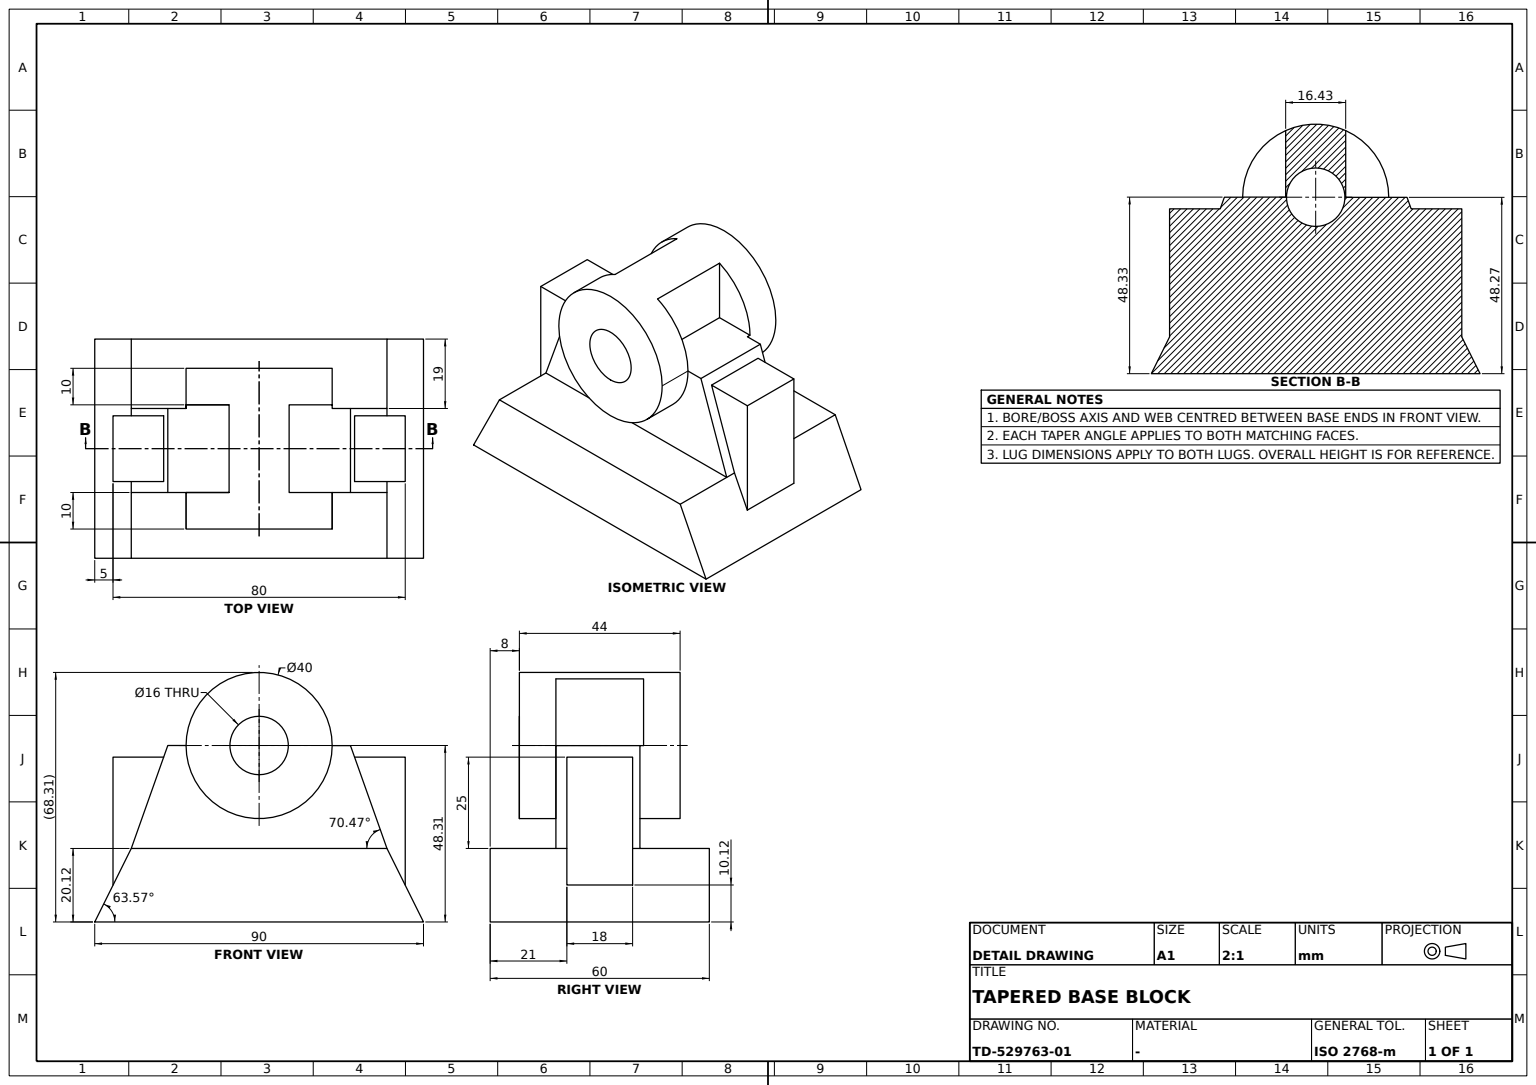
ISO-10303-21;
HEADER;
FILE_DESCRIPTION((''),'2;1');
FILE_NAME('','',(''),(''),'','','');
FILE_SCHEMA(('AUTOMOTIVE_DESIGN'));
ENDSEC;
DATA;
#1=APPLICATION_CONTEXT('');
#2=PRODUCT_CONTEXT('',#1,'mechanical');
#3=PRODUCT('','','',(#2));
#4=PRODUCT_DEFINITION_FORMATION('','',#3);
#5=PRODUCT_DEFINITION_CONTEXT('',#1,'design');
#6=PRODUCT_DEFINITION('','',#4,#5);
#7=PRODUCT_DEFINITION_SHAPE('','',#6);
#8=(LENGTH_UNIT()NAMED_UNIT(*)SI_UNIT(.MILLI.,.METRE.));
#9=(NAMED_UNIT(*)PLANE_ANGLE_UNIT()SI_UNIT($,.RADIAN.));
#10=(NAMED_UNIT(*)SI_UNIT($,.STERADIAN.)SOLID_ANGLE_UNIT());
#11=UNCERTAINTY_MEASURE_WITH_UNIT(LENGTH_MEASURE(0.005),#8,'distance_accuracy_value','');
#12=(GEOMETRIC_REPRESENTATION_CONTEXT(3)GLOBAL_UNCERTAINTY_ASSIGNED_CONTEXT((#11))GLOBAL_UNIT_ASSIGNED_CONTEXT((#8,#9,#10))REPRESENTATION_CONTEXT('',''));
#13=CARTESIAN_POINT('',(9.,71.13019,45.122224));
#14=VERTEX_POINT('',#13);
#15=CARTESIAN_POINT('',(9.,80.,20.122224));
#16=VERTEX_POINT('',#15);
#17=DIRECTION('',(0.,0.334371072,-0.942441503));
#18=VECTOR('',#17,1000.);
#19=LINE('',#15,#18);
#20=EDGE_CURVE('',#14,#16,#19,.T.);
#21=ORIENTED_EDGE('',*,*,#20,.F.);
#22=CARTESIAN_POINT('',(-9.,71.13019,45.122224));
#23=VERTEX_POINT('',#22);
#24=CARTESIAN_POINT('',(11.,71.13019,45.122224));
#25=DIRECTION('',(1.,0.,0.));
#26=VECTOR('',#25,1000.);
#27=LINE('',#24,#26);
#28=EDGE_CURVE('',#23,#14,#27,.T.);
#29=ORIENTED_EDGE('',*,*,#28,.F.);
#30=CARTESIAN_POINT('',(-9.,80.,20.122224));
#31=VERTEX_POINT('',#30);
#32=CARTESIAN_POINT('',(-9.,80.55902,18.546598));
#33=LINE('',#32,#18);
#34=EDGE_CURVE('',#23,#31,#33,.T.);
#35=ORIENTED_EDGE('',*,*,#34,.T.);
#36=CARTESIAN_POINT('',(-11.,80.,20.122224));
#37=VERTEX_POINT('',#36);
#38=CARTESIAN_POINT('',(11.,80.,20.122224));
#39=LINE('',#38,#26);
#40=EDGE_CURVE('',#37,#31,#39,.T.);
#41=ORIENTED_EDGE('',*,*,#40,.F.);
#42=CARTESIAN_POINT('',(-11.,70.012761,48.271755));
#43=VERTEX_POINT('',#42);
#44=CARTESIAN_POINT('',(-11.,77.396698,27.459759));
#45=DIRECTION('',(0.,-0.334371072,0.942441503));
#46=VECTOR('',#45,1000.);
#47=LINE('',#44,#46);
#48=EDGE_CURVE('',#37,#43,#47,.T.);
#49=ORIENTED_EDGE('',*,*,#48,.T.);
#50=CARTESIAN_POINT('',(12.,70.012761,48.271755));
#51=VERTEX_POINT('',#50);
#52=CARTESIAN_POINT('',(11.,70.012761,48.271755));
#53=DIRECTION('',(-1.,0.,0.));
#54=VECTOR('',#53,1000.);
#55=LINE('',#52,#54);
#56=EDGE_CURVE('',#51,#43,#55,.T.);
#57=ORIENTED_EDGE('',*,*,#56,.F.);
#58=CARTESIAN_POINT('',(12.,80.,20.122224));
#59=VERTEX_POINT('',#58);
#60=CARTESIAN_POINT('',(12.,77.396698,27.459759));
#61=LINE('',#60,#46);
#62=EDGE_CURVE('',#59,#51,#61,.T.);
#63=ORIENTED_EDGE('',*,*,#62,.F.);
#64=EDGE_CURVE('',#16,#59,#39,.T.);
#65=ORIENTED_EDGE('',*,*,#64,.F.);
#66=EDGE_LOOP('',(#21,#29,#35,#41,#49,#57,#63,#65));
#67=FACE_BOUND('',#66,.T.);
#68=DIRECTION('',(0.,0.942441503,0.334371072));
#69=AXIS2_PLACEMENT_3D('',#38,#68,#45);
#70=PLANE('',#69);
#71=ADVANCED_FACE('',(#67),#70,.T.);
#72=CARTESIAN_POINT('',(12.,36.78216,66.536631));
#73=VERTEX_POINT('',#72);
#74=CARTESIAN_POINT('',(12.,25.000016,48.315907));
#75=VERTEX_POINT('',#74);
#76=CARTESIAN_POINT('',(12.,45.,48.307722));
#77=DIRECTION('',(0.,0.,-1.));
#78=AXIS2_PLACEMENT_3D('',#76,#25,#77);
#79=CIRCLE('',#78,20.);
#80=EDGE_CURVE('',#73,#75,#79,.T.);
#81=ORIENTED_EDGE('',*,*,#80,.T.);
#82=CARTESIAN_POINT('',(22.,25.000001,48.302951));
#83=VERTEX_POINT('',#82);
#84=CARTESIAN_POINT('',(12.,25.000001,48.302951));
#85=LINE('',#84,#26);
#86=EDGE_CURVE('',#75,#83,#85,.T.);
#87=ORIENTED_EDGE('',*,*,#86,.T.);
#88=CARTESIAN_POINT('',(22.,65.,48.296679));
#89=VERTEX_POINT('',#88);
#90=CARTESIAN_POINT('',(22.,45.,48.307722));
#91=AXIS2_PLACEMENT_3D('',#90,#25,#77);
#92=CIRCLE('',#91,20.);
#93=EDGE_CURVE('',#89,#83,#92,.T.);
#94=ORIENTED_EDGE('',*,*,#93,.F.);
#95=CARTESIAN_POINT('',(12.,64.999991,48.284967));
#96=VERTEX_POINT('',#95);
#97=CARTESIAN_POINT('',(12.,65.,48.29818));
#98=CARTESIAN_POINT('',(15.333333,65.,48.29818));
#99=CARTESIAN_POINT('',(18.666667,65.,48.29818));
#100=CARTESIAN_POINT('',(22.,65.,48.29818));
#101=B_SPLINE_CURVE_WITH_KNOTS('',3,(#97,#98,#99,#100),.UNSPECIFIED.,.F.,.F.,(4,4),(-5.,4.999999833),.UNSPECIFIED.);
#102=EDGE_CURVE('',#89,#96,#101,.F.);
#103=ORIENTED_EDGE('',*,*,#102,.T.);
#104=CARTESIAN_POINT('',(12.,53.214887,66.537961));
#105=VERTEX_POINT('',#104);
#106=EDGE_CURVE('',#96,#105,#79,.T.);
#107=ORIENTED_EDGE('',*,*,#106,.T.);
#108=CARTESIAN_POINT('',(-12.,53.214888,66.542733));
#109=VERTEX_POINT('',#108);
#110=CARTESIAN_POINT('',(12.,53.214887,66.542733));
#111=LINE('',#110,#26);
#112=EDGE_CURVE('',#105,#109,#111,.F.);
#113=ORIENTED_EDGE('',*,*,#112,.T.);
#114=CARTESIAN_POINT('',(-12.,64.999984,48.289738));
#115=VERTEX_POINT('',#114);
#116=CARTESIAN_POINT('',(-12.,45.,48.307722));
#117=DIRECTION('',(0.,0.,1.));
#118=AXIS2_PLACEMENT_3D('',#116,#53,#117);
#119=CIRCLE('',#118,20.);
#120=EDGE_CURVE('',#109,#115,#119,.T.);
#121=ORIENTED_EDGE('',*,*,#120,.T.);
#122=CARTESIAN_POINT('',(-11.,64.999968,48.271755));
#123=VERTEX_POINT('',#122);
#124=CARTESIAN_POINT('',(-12.,64.999968,48.271755));
#125=LINE('',#124,#26);
#126=EDGE_CURVE('',#115,#123,#125,.T.);
#127=ORIENTED_EDGE('',*,*,#126,.T.);
#128=CARTESIAN_POINT('',(-11.,25.000008,48.320677));
#129=VERTEX_POINT('',#128);
#130=CARTESIAN_POINT('',(-11.,45.,48.307722));
#131=AXIS2_PLACEMENT_3D('',#130,#25,#77);
#132=CIRCLE('',#131,20.);
#133=EDGE_CURVE('',#129,#123,#132,.T.);
#134=ORIENTED_EDGE('',*,*,#133,.F.);
#135=CARTESIAN_POINT('',(-12.,25.000008,48.320678));
#136=VERTEX_POINT('',#135);
#137=CARTESIAN_POINT('',(-12.,25.000017,48.333633));
#138=LINE('',#137,#26);
#139=EDGE_CURVE('',#136,#129,#138,.T.);
#140=ORIENTED_EDGE('',*,*,#139,.F.);
#141=CARTESIAN_POINT('',(-12.,36.78216,66.541402));
#142=VERTEX_POINT('',#141);
#143=EDGE_CURVE('',#136,#142,#119,.T.);
#144=ORIENTED_EDGE('',*,*,#143,.T.);
#145=CARTESIAN_POINT('',(12.,36.78216,66.541402));
#146=LINE('',#145,#26);
#147=EDGE_CURVE('',#73,#142,#146,.F.);
#148=ORIENTED_EDGE('',*,*,#147,.F.);
#149=EDGE_LOOP('',(#81,#87,#94,#103,#107,#113,#121,#127,#134,#140,#144,#148));
#150=FACE_BOUND('',#149,.T.);
#151=CARTESIAN_POINT('',(-22.,45.,28.307722));
#152=VERTEX_POINT('',#151);
#153=CARTESIAN_POINT('',(-22.,45.,48.307722));
#154=AXIS2_PLACEMENT_3D('',#153,#25,#77);
#155=CIRCLE('',#154,20.);
#156=EDGE_CURVE('',#152,#152,#155,.F.);
#157=ORIENTED_EDGE('',*,*,#156,.F.);
#158=EDGE_LOOP('',(#157));
#159=FACE_BOUND('',#158,.T.);
#160=CARTESIAN_POINT('',(17.,45.,48.307722));
#161=DIRECTION('',(0.,1.,0.));
#162=AXIS2_PLACEMENT_3D('',#160,#25,#161);
#163=CYLINDRICAL_SURFACE('',#162,20.);
#164=ADVANCED_FACE('',(#150,#159),#163,.T.);
#165=CARTESIAN_POINT('',(12.,45.,48.29818));
#166=AXIS2_PLACEMENT_3D('',#165,#25,#77);
#167=CIRCLE('',#166,20.);
#168=EDGE_CURVE('',#75,#96,#167,.T.);
#169=ORIENTED_EDGE('',*,*,#168,.T.);
#170=ORIENTED_EDGE('',*,*,#102,.F.);
#171=CARTESIAN_POINT('',(22.,45.,48.29818));
#172=AXIS2_PLACEMENT_3D('',#171,#25,#77);
#173=CIRCLE('',#172,20.);
#174=EDGE_CURVE('',#83,#89,#173,.T.);
#175=ORIENTED_EDGE('',*,*,#174,.F.);
#176=ORIENTED_EDGE('',*,*,#86,.F.);
#177=EDGE_LOOP('',(#169,#170,#175,#176));
#178=FACE_BOUND('',#177,.T.);
#179=CARTESIAN_POINT('',(17.,45.,48.29818));
#180=AXIS2_PLACEMENT_3D('',#179,#25,#161);
#181=CYLINDRICAL_SURFACE('',#180,20.);
#182=ADVANCED_FACE('',(#178),#181,.T.);
#183=CARTESIAN_POINT('',(-30.,0.,0.));
#184=VERTEX_POINT('',#183);
#185=CARTESIAN_POINT('',(30.,0.,0.));
#186=VERTEX_POINT('',#185);
#187=CARTESIAN_POINT('',(0.,0.,0.));
#188=LINE('',#187,#26);
#189=EDGE_CURVE('',#184,#186,#188,.T.);
#190=ORIENTED_EDGE('',*,*,#189,.F.);
#191=CARTESIAN_POINT('',(-30.,90.,0.));
#192=VERTEX_POINT('',#191);
#193=VECTOR('',#161,1000.);
#194=LINE('',#183,#193);
#195=EDGE_CURVE('',#184,#192,#194,.T.);
#196=ORIENTED_EDGE('',*,*,#195,.T.);
#197=CARTESIAN_POINT('',(30.,90.,0.));
#198=VERTEX_POINT('',#197);
#199=CARTESIAN_POINT('',(0.,90.,0.));
#200=LINE('',#199,#26);
#201=EDGE_CURVE('',#192,#198,#200,.T.);
#202=ORIENTED_EDGE('',*,*,#201,.T.);
#203=LINE('',#185,#193);
#204=EDGE_CURVE('',#186,#198,#203,.T.);
#205=ORIENTED_EDGE('',*,*,#204,.F.);
#206=EDGE_LOOP('',(#190,#196,#202,#205));
#207=FACE_BOUND('',#206,.T.);
#208=AXIS2_PLACEMENT_3D('',#187,#77,#161);
#209=PLANE('',#208);
#210=ADVANCED_FACE('',(#207),#209,.T.);
#211=CARTESIAN_POINT('',(-30.,80.,20.122224));
#212=VERTEX_POINT('',#211);
#213=CARTESIAN_POINT('',(0.,80.,20.122224));
#214=LINE('',#213,#26);
#215=EDGE_CURVE('',#212,#37,#214,.T.);
#216=ORIENTED_EDGE('',*,*,#215,.F.);
#217=CARTESIAN_POINT('',(-30.,10.,20.122224));
#218=VERTEX_POINT('',#217);
#219=CARTESIAN_POINT('',(-30.,0.,20.122224));
#220=DIRECTION('',(0.,-1.,0.));
#221=VECTOR('',#220,1000.);
#222=LINE('',#219,#221);
#223=EDGE_CURVE('',#212,#218,#222,.T.);
#224=ORIENTED_EDGE('',*,*,#223,.T.);
#225=CARTESIAN_POINT('',(-11.,10.,20.122224));
#226=VERTEX_POINT('',#225);
#227=CARTESIAN_POINT('',(0.,10.,20.122224));
#228=LINE('',#227,#26);
#229=EDGE_CURVE('',#218,#226,#228,.T.);
#230=ORIENTED_EDGE('',*,*,#229,.T.);
#231=LINE('',#36,#193);
#232=EDGE_CURVE('',#226,#37,#231,.T.);
#233=ORIENTED_EDGE('',*,*,#232,.T.);
#234=EDGE_LOOP('',(#216,#224,#230,#233));
#235=FACE_BOUND('',#234,.T.);
#236=AXIS2_PLACEMENT_3D('',#213,#117,#220);
#237=PLANE('',#236);
#238=ADVANCED_FACE('',(#235),#237,.T.);
#239=CARTESIAN_POINT('',(30.,80.,20.122224));
#240=VERTEX_POINT('',#239);
#241=CARTESIAN_POINT('',(30.,10.,20.122224));
#242=VERTEX_POINT('',#241);
#243=CARTESIAN_POINT('',(30.,0.,20.122224));
#244=LINE('',#243,#221);
#245=EDGE_CURVE('',#240,#242,#244,.T.);
#246=ORIENTED_EDGE('',*,*,#245,.F.);
#247=EDGE_CURVE('',#59,#240,#214,.T.);
#248=ORIENTED_EDGE('',*,*,#247,.F.);
#249=CARTESIAN_POINT('',(12.,10.,20.122224));
#250=VERTEX_POINT('',#249);
#251=LINE('',#58,#193);
#252=EDGE_CURVE('',#250,#59,#251,.T.);
#253=ORIENTED_EDGE('',*,*,#252,.F.);
#254=EDGE_CURVE('',#250,#242,#228,.T.);
#255=ORIENTED_EDGE('',*,*,#254,.T.);
#256=EDGE_LOOP('',(#246,#248,#253,#255));
#257=FACE_BOUND('',#256,.T.);
#258=ADVANCED_FACE('',(#257),#237,.T.);
#259=CARTESIAN_POINT('',(-9.,84.984815,10.122125));
#260=VERTEX_POINT('',#259);
#261=CARTESIAN_POINT('',(-9.,85.,45.122224));
#262=VERTEX_POINT('',#261);
#263=CARTESIAN_POINT('',(-9.,85.,20.122224));
#264=VECTOR('',#117,1000.);
#265=LINE('',#263,#264);
#266=EDGE_CURVE('',#260,#262,#265,.T.);
#267=ORIENTED_EDGE('',*,*,#266,.T.);
#268=CARTESIAN_POINT('',(9.,85.,45.122224));
#269=VERTEX_POINT('',#268);
#270=CARTESIAN_POINT('',(0.,85.,45.122224));
#271=LINE('',#270,#26);
#272=EDGE_CURVE('',#262,#269,#271,.T.);
#273=ORIENTED_EDGE('',*,*,#272,.T.);
#274=CARTESIAN_POINT('',(9.,84.984815,10.122125));
#275=VERTEX_POINT('',#274);
#276=CARTESIAN_POINT('',(9.,85.,20.122224));
#277=LINE('',#276,#264);
#278=EDGE_CURVE('',#275,#269,#277,.T.);
#279=ORIENTED_EDGE('',*,*,#278,.F.);
#280=CARTESIAN_POINT('',(-9.,84.96963,10.122224));
#281=CARTESIAN_POINT('',(-3.,84.96963,10.122224));
#282=CARTESIAN_POINT('',(3.,84.96963,10.122224));
#283=CARTESIAN_POINT('',(9.,84.96963,10.122224));
#284=B_SPLINE_CURVE_WITH_KNOTS('',3,(#280,#281,#282,#283),.UNSPECIFIED.,.F.,.F.,(4,4),(-8.99999975,8.99999975),.UNSPECIFIED.);
#285=EDGE_CURVE('',#260,#275,#284,.T.);
#286=ORIENTED_EDGE('',*,*,#285,.F.);
#287=EDGE_LOOP('',(#267,#273,#279,#286));
#288=FACE_BOUND('',#287,.T.);
#289=AXIS2_PLACEMENT_3D('',#263,#220,#25);
#290=PLANE('',#289);
#291=ADVANCED_FACE('',(#288),#290,.F.);
#292=CARTESIAN_POINT('',(9.,5.,45.122224));
#293=VERTEX_POINT('',#292);
#294=CARTESIAN_POINT('',(9.,18.86981,45.122224));
#295=VERTEX_POINT('',#294);
#296=CARTESIAN_POINT('',(9.,0.,45.122224));
#297=LINE('',#296,#193);
#298=EDGE_CURVE('',#293,#295,#297,.T.);
#299=ORIENTED_EDGE('',*,*,#298,.F.);
#300=CARTESIAN_POINT('',(9.,5.015185,10.122124));
#301=VERTEX_POINT('',#300);
#302=CARTESIAN_POINT('',(9.,5.,20.122224));
#303=LINE('',#302,#264);
#304=EDGE_CURVE('',#301,#293,#303,.T.);
#305=ORIENTED_EDGE('',*,*,#304,.F.);
#306=CARTESIAN_POINT('',(9.,10.,20.122224));
#307=VERTEX_POINT('',#306);
#308=CARTESIAN_POINT('',(9.,9.009713,18.129546));
#309=DIRECTION('',(0.,-0.445036504,-0.895512429));
#310=VECTOR('',#309,1000.);
#311=LINE('',#308,#310);
#312=EDGE_CURVE('',#307,#301,#311,.T.);
#313=ORIENTED_EDGE('',*,*,#312,.F.);
#314=CARTESIAN_POINT('',(9.,9.44098,18.546598));
#315=DIRECTION('',(0.,-0.334371072,-0.942441503));
#316=VECTOR('',#315,1000.);
#317=LINE('',#314,#316);
#318=EDGE_CURVE('',#295,#307,#317,.T.);
#319=ORIENTED_EDGE('',*,*,#318,.F.);
#320=EDGE_LOOP('',(#299,#305,#313,#319));
#321=FACE_BOUND('',#320,.T.);
#322=AXIS2_PLACEMENT_3D('',#302,#25,#161);
#323=PLANE('',#322);
#324=ADVANCED_FACE('',(#321),#323,.T.);
#325=ORIENTED_EDGE('',*,*,#189,.T.);
#326=LINE('',#185,#310);
#327=EDGE_CURVE('',#242,#186,#326,.T.);
#328=ORIENTED_EDGE('',*,*,#327,.F.);
#329=ORIENTED_EDGE('',*,*,#254,.F.);
#330=EDGE_CURVE('',#307,#250,#228,.T.);
#331=ORIENTED_EDGE('',*,*,#330,.F.);
#332=ORIENTED_EDGE('',*,*,#312,.T.);
#333=CARTESIAN_POINT('',(-9.,5.015185,10.122124));
#334=VERTEX_POINT('',#333);
#335=CARTESIAN_POINT('',(-9.,5.,10.122224));
#336=CARTESIAN_POINT('',(-3.,5.,10.122224));
#337=CARTESIAN_POINT('',(3.,5.,10.122224));
#338=CARTESIAN_POINT('',(9.,5.,10.122224));
#339=B_SPLINE_CURVE_WITH_KNOTS('',3,(#335,#336,#337,#338),.UNSPECIFIED.,.F.,.F.,(4,4),(0.00000025,17.99999975),.UNSPECIFIED.);
#340=EDGE_CURVE('',#334,#301,#339,.T.);
#341=ORIENTED_EDGE('',*,*,#340,.F.);
#342=CARTESIAN_POINT('',(-9.,10.,20.122224));
#343=VERTEX_POINT('',#342);
#344=LINE('',#342,#310);
#345=EDGE_CURVE('',#343,#334,#344,.T.);
#346=ORIENTED_EDGE('',*,*,#345,.F.);
#347=EDGE_CURVE('',#226,#343,#228,.T.);
#348=ORIENTED_EDGE('',*,*,#347,.F.);
#349=ORIENTED_EDGE('',*,*,#229,.F.);
#350=LINE('',#183,#310);
#351=EDGE_CURVE('',#218,#184,#350,.T.);
#352=ORIENTED_EDGE('',*,*,#351,.T.);
#353=EDGE_LOOP('',(#325,#328,#329,#331,#332,#341,#346,#348,#349,#352));
#354=FACE_BOUND('',#353,.T.);
#355=DIRECTION('',(0.,-0.895512429,0.445036504));
#356=AXIS2_PLACEMENT_3D('',#227,#355,#309);
#357=PLANE('',#356);
#358=ADVANCED_FACE('',(#354),#357,.T.);
#359=CARTESIAN_POINT('',(12.,53.214887,48.271755));
#360=VERTEX_POINT('',#359);
#361=CARTESIAN_POINT('',(12.,53.214887,67.271755));
#362=VECTOR('',#77,1000.);
#363=LINE('',#361,#362);
#364=EDGE_CURVE('',#105,#360,#363,.T.);
#365=ORIENTED_EDGE('',*,*,#364,.F.);
#366=ORIENTED_EDGE('',*,*,#106,.F.);
#367=CARTESIAN_POINT('',(12.,0.,48.271755));
#368=LINE('',#367,#193);
#369=EDGE_CURVE('',#360,#96,#368,.T.);
#370=ORIENTED_EDGE('',*,*,#369,.F.);
#371=EDGE_LOOP('',(#365,#366,#370));
#372=FACE_BOUND('',#371,.T.);
#373=CARTESIAN_POINT('',(12.,0.,0.));
#374=AXIS2_PLACEMENT_3D('',#373,#25,#161);
#375=PLANE('',#374);
#376=ADVANCED_FACE('',(#372),#375,.F.);
#377=CARTESIAN_POINT('',(30.,72.174826,35.868215));
#378=DIRECTION('',(0.,-0.445036504,0.895512429));
#379=VECTOR('',#378,1000.);
#380=LINE('',#377,#379);
#381=EDGE_CURVE('',#198,#240,#380,.T.);
#382=ORIENTED_EDGE('',*,*,#381,.T.);
#383=ORIENTED_EDGE('',*,*,#245,.T.);
#384=ORIENTED_EDGE('',*,*,#327,.T.);
#385=ORIENTED_EDGE('',*,*,#204,.T.);
#386=EDGE_LOOP('',(#382,#383,#384,#385));
#387=FACE_BOUND('',#386,.T.);
#388=AXIS2_PLACEMENT_3D('',#185,#25,#161);
#389=PLANE('',#388);
#390=ADVANCED_FACE('',(#387),#389,.T.);
#391=ORIENTED_EDGE('',*,*,#120,.F.);
#392=CARTESIAN_POINT('',(-12.,53.214887,48.271755));
#393=VERTEX_POINT('',#392);
#394=CARTESIAN_POINT('',(-12.,53.214887,0.));
#395=LINE('',#394,#362);
#396=EDGE_CURVE('',#109,#393,#395,.T.);
#397=ORIENTED_EDGE('',*,*,#396,.T.);
#398=CARTESIAN_POINT('',(-12.,70.214887,48.271755));
#399=LINE('',#398,#193);
#400=EDGE_CURVE('',#393,#115,#399,.T.);
#401=ORIENTED_EDGE('',*,*,#400,.T.);
#402=EDGE_LOOP('',(#391,#397,#401));
#403=FACE_BOUND('',#402,.T.);
#404=CARTESIAN_POINT('',(-12.,0.,0.));
#405=AXIS2_PLACEMENT_3D('',#404,#53,#220);
#406=PLANE('',#405);
#407=ADVANCED_FACE('',(#403),#406,.F.);
#408=CARTESIAN_POINT('',(-12.,36.78216,48.333633));
#409=VERTEX_POINT('',#408);
#410=CARTESIAN_POINT('',(-12.,36.78216,0.));
#411=LINE('',#410,#362);
#412=EDGE_CURVE('',#142,#409,#411,.T.);
#413=ORIENTED_EDGE('',*,*,#412,.T.);
#414=CARTESIAN_POINT('',(12.,36.78216,48.333633));
#415=VERTEX_POINT('',#414);
#416=CARTESIAN_POINT('',(22.,36.78216,48.333633));
#417=LINE('',#416,#54);
#418=EDGE_CURVE('',#415,#409,#417,.T.);
#419=ORIENTED_EDGE('',*,*,#418,.F.);
#420=CARTESIAN_POINT('',(12.,36.78216,67.333633));
#421=LINE('',#420,#362);
#422=EDGE_CURVE('',#73,#415,#421,.T.);
#423=ORIENTED_EDGE('',*,*,#422,.F.);
#424=ORIENTED_EDGE('',*,*,#147,.T.);
#425=EDGE_LOOP('',(#413,#419,#423,#424));
#426=FACE_BOUND('',#425,.T.);
#427=CARTESIAN_POINT('',(22.,36.78216,67.333633));
#428=AXIS2_PLACEMENT_3D('',#427,#161,#77);
#429=PLANE('',#428);
#430=ADVANCED_FACE('',(#426),#429,.F.);
#431=CARTESIAN_POINT('',(-12.,0.,48.333633));
#432=LINE('',#431,#193);
#433=EDGE_CURVE('',#136,#409,#432,.T.);
#434=ORIENTED_EDGE('',*,*,#433,.T.);
#435=ORIENTED_EDGE('',*,*,#412,.F.);
#436=ORIENTED_EDGE('',*,*,#143,.F.);
#437=EDGE_LOOP('',(#434,#435,#436));
#438=FACE_BOUND('',#437,.T.);
#439=ADVANCED_FACE('',(#438),#406,.F.);
#440=ORIENTED_EDGE('',*,*,#156,.T.);
#441=EDGE_LOOP('',(#440));
#442=FACE_BOUND('',#441,.T.);
#443=CARTESIAN_POINT('',(-22.,45.,40.307722));
#444=VERTEX_POINT('',#443);
#445=CIRCLE('',#154,8.);
#446=EDGE_CURVE('',#444,#444,#445,.T.);
#447=ORIENTED_EDGE('',*,*,#446,.T.);
#448=EDGE_LOOP('',(#447));
#449=FACE_BOUND('',#448,.T.);
#450=CARTESIAN_POINT('',(-22.,0.,0.));
#451=AXIS2_PLACEMENT_3D('',#450,#25,#161);
#452=PLANE('',#451);
#453=ADVANCED_FACE('',(#442,#449),#452,.F.);
#454=CARTESIAN_POINT('',(-9.,18.86981,45.122224));
#455=VERTEX_POINT('',#454);
#456=CARTESIAN_POINT('',(0.,18.86981,45.122224));
#457=LINE('',#456,#26);
#458=EDGE_CURVE('',#455,#295,#457,.T.);
#459=ORIENTED_EDGE('',*,*,#458,.F.);
#460=CARTESIAN_POINT('',(-9.,5.,45.122224));
#461=VERTEX_POINT('',#460);
#462=CARTESIAN_POINT('',(-9.,0.,45.122224));
#463=LINE('',#462,#221);
#464=EDGE_CURVE('',#455,#461,#463,.T.);
#465=ORIENTED_EDGE('',*,*,#464,.T.);
#466=CARTESIAN_POINT('',(0.,5.,45.122224));
#467=LINE('',#466,#54);
#468=EDGE_CURVE('',#293,#461,#467,.T.);
#469=ORIENTED_EDGE('',*,*,#468,.F.);
#470=ORIENTED_EDGE('',*,*,#298,.T.);
#471=EDGE_LOOP('',(#459,#465,#469,#470));
#472=FACE_BOUND('',#471,.T.);
#473=CARTESIAN_POINT('',(0.,0.,45.122224));
#474=AXIS2_PLACEMENT_3D('',#473,#117,#25);
#475=PLANE('',#474);
#476=ADVANCED_FACE('',(#472),#475,.T.);
#477=CARTESIAN_POINT('',(12.,70.214887,48.271755));
#478=LINE('',#477,#221);
#479=EDGE_CURVE('',#51,#96,#478,.T.);
#480=ORIENTED_EDGE('',*,*,#479,.T.);
#481=ORIENTED_EDGE('',*,*,#168,.F.);
#482=CARTESIAN_POINT('',(12.,20.,48.307722));
#483=VERTEX_POINT('',#482);
#484=CARTESIAN_POINT('',(12.,0.,48.307722));
#485=LINE('',#484,#221);
#486=EDGE_CURVE('',#75,#483,#485,.T.);
#487=ORIENTED_EDGE('',*,*,#486,.T.);
#488=CARTESIAN_POINT('',(12.,2.54094,-0.901506));
#489=LINE('',#488,#316);
#490=EDGE_CURVE('',#483,#250,#489,.T.);
#491=ORIENTED_EDGE('',*,*,#490,.T.);
#492=ORIENTED_EDGE('',*,*,#252,.T.);
#493=ORIENTED_EDGE('',*,*,#62,.T.);
#494=EDGE_LOOP('',(#480,#481,#487,#491,#492,#493));
#495=FACE_BOUND('',#494,.T.);
#496=ADVANCED_FACE('',(#495),#375,.T.);
#497=CARTESIAN_POINT('',(-11.,25.000017,48.333633));
#498=CARTESIAN_POINT('',(-3.333333,25.000017,48.333633));
#499=CARTESIAN_POINT('',(4.333333,25.000017,48.333633));
#500=CARTESIAN_POINT('',(12.,25.000017,48.333633));
#501=B_SPLINE_CURVE_WITH_KNOTS('',3,(#497,#498,#499,#500),.UNSPECIFIED.,.F.,.F.,(4,4),(11.,34.),.UNSPECIFIED.);
#502=EDGE_CURVE('',#129,#75,#501,.T.);
#503=ORIENTED_EDGE('',*,*,#502,.T.);
#504=CARTESIAN_POINT('',(12.,19.78216,48.333633));
#505=LINE('',#504,#193);
#506=EDGE_CURVE('',#75,#415,#505,.T.);
#507=ORIENTED_EDGE('',*,*,#506,.T.);
#508=ORIENTED_EDGE('',*,*,#418,.T.);
#509=ORIENTED_EDGE('',*,*,#433,.F.);
#510=ORIENTED_EDGE('',*,*,#139,.T.);
#511=EDGE_LOOP('',(#503,#507,#508,#509,#510));
#512=FACE_BOUND('',#511,.T.);
#513=CARTESIAN_POINT('',(22.,19.78216,48.333633));
#514=AXIS2_PLACEMENT_3D('',#513,#117,#161);
#515=PLANE('',#514);
#516=ADVANCED_FACE('',(#512),#515,.T.);
#517=CARTESIAN_POINT('',(-11.,20.,48.307722));
#518=VERTEX_POINT('',#517);
#519=CARTESIAN_POINT('',(-11.,0.,48.307722));
#520=LINE('',#519,#221);
#521=EDGE_CURVE('',#129,#518,#520,.T.);
#522=ORIENTED_EDGE('',*,*,#521,.F.);
#523=ORIENTED_EDGE('',*,*,#133,.T.);
#524=CARTESIAN_POINT('',(-11.,70.214887,48.271755));
#525=LINE('',#524,#221);
#526=EDGE_CURVE('',#43,#123,#525,.T.);
#527=ORIENTED_EDGE('',*,*,#526,.F.);
#528=ORIENTED_EDGE('',*,*,#48,.F.);
#529=ORIENTED_EDGE('',*,*,#232,.F.);
#530=CARTESIAN_POINT('',(-11.,2.54094,-0.901506));
#531=LINE('',#530,#316);
#532=EDGE_CURVE('',#518,#226,#531,.T.);
#533=ORIENTED_EDGE('',*,*,#532,.F.);
#534=EDGE_LOOP('',(#522,#523,#527,#528,#529,#533));
#535=FACE_BOUND('',#534,.T.);
#536=CARTESIAN_POINT('',(-11.,0.,0.));
#537=AXIS2_PLACEMENT_3D('',#536,#25,#161);
#538=PLANE('',#537);
#539=ADVANCED_FACE('',(#535),#538,.F.);
#540=CARTESIAN_POINT('',(9.,90.,0.));
#541=DIRECTION('',(0.,0.445036504,-0.895512429));
#542=VECTOR('',#541,1000.);
#543=LINE('',#540,#542);
#544=EDGE_CURVE('',#16,#275,#543,.T.);
#545=ORIENTED_EDGE('',*,*,#544,.T.);
#546=ORIENTED_EDGE('',*,*,#278,.T.);
#547=EDGE_CURVE('',#14,#269,#297,.T.);
#548=ORIENTED_EDGE('',*,*,#547,.F.);
#549=ORIENTED_EDGE('',*,*,#20,.T.);
#550=EDGE_LOOP('',(#545,#546,#548,#549));
#551=FACE_BOUND('',#550,.T.);
#552=ADVANCED_FACE('',(#551),#323,.T.);
#553=ORIENTED_EDGE('',*,*,#351,.F.);
#554=ORIENTED_EDGE('',*,*,#223,.F.);
#555=CARTESIAN_POINT('',(-30.,72.174826,35.868215));
#556=LINE('',#555,#379);
#557=EDGE_CURVE('',#192,#212,#556,.T.);
#558=ORIENTED_EDGE('',*,*,#557,.F.);
#559=ORIENTED_EDGE('',*,*,#195,.F.);
#560=EDGE_LOOP('',(#553,#554,#558,#559));
#561=FACE_BOUND('',#560,.T.);
#562=AXIS2_PLACEMENT_3D('',#183,#25,#161);
#563=PLANE('',#562);
#564=ADVANCED_FACE('',(#561),#563,.F.);
#565=ORIENTED_EDGE('',*,*,#174,.T.);
#566=ORIENTED_EDGE('',*,*,#93,.T.);
#567=EDGE_LOOP('',(#565,#566));
#568=FACE_BOUND('',#567,.T.);
#569=CARTESIAN_POINT('',(22.,45.,40.307722));
#570=VERTEX_POINT('',#569);
#571=CIRCLE('',#91,8.);
#572=EDGE_CURVE('',#570,#570,#571,.T.);
#573=ORIENTED_EDGE('',*,*,#572,.F.);
#574=EDGE_LOOP('',(#573));
#575=FACE_BOUND('',#574,.T.);
#576=CARTESIAN_POINT('',(22.,0.,0.));
#577=AXIS2_PLACEMENT_3D('',#576,#25,#161);
#578=PLANE('',#577);
#579=ADVANCED_FACE('',(#568,#575),#578,.T.);
#580=CARTESIAN_POINT('',(-9.,5.,20.122224));
#581=LINE('',#580,#264);
#582=EDGE_CURVE('',#334,#461,#581,.T.);
#583=ORIENTED_EDGE('',*,*,#582,.T.);
#584=ORIENTED_EDGE('',*,*,#464,.F.);
#585=CARTESIAN_POINT('',(-9.,20.,48.307722));
#586=LINE('',#585,#316);
#587=EDGE_CURVE('',#455,#343,#586,.T.);
#588=ORIENTED_EDGE('',*,*,#587,.T.);
#589=ORIENTED_EDGE('',*,*,#345,.T.);
#590=EDGE_LOOP('',(#583,#584,#588,#589));
#591=FACE_BOUND('',#590,.T.);
#592=AXIS2_PLACEMENT_3D('',#263,#53,#220);
#593=PLANE('',#592);
#594=ADVANCED_FACE('',(#591),#593,.T.);
#595=ORIENTED_EDGE('',*,*,#468,.T.);
#596=ORIENTED_EDGE('',*,*,#582,.F.);
#597=ORIENTED_EDGE('',*,*,#340,.T.);
#598=ORIENTED_EDGE('',*,*,#304,.T.);
#599=EDGE_LOOP('',(#595,#596,#597,#598));
#600=FACE_BOUND('',#599,.T.);
#601=AXIS2_PLACEMENT_3D('',#302,#161,#53);
#602=PLANE('',#601);
#603=ADVANCED_FACE('',(#600),#602,.F.);
#604=ORIENTED_EDGE('',*,*,#272,.F.);
#605=EDGE_CURVE('',#262,#23,#463,.T.);
#606=ORIENTED_EDGE('',*,*,#605,.T.);
#607=ORIENTED_EDGE('',*,*,#28,.T.);
#608=ORIENTED_EDGE('',*,*,#547,.T.);
#609=EDGE_LOOP('',(#604,#606,#607,#608));
#610=FACE_BOUND('',#609,.T.);
#611=ADVANCED_FACE('',(#610),#475,.T.);
#612=ORIENTED_EDGE('',*,*,#486,.F.);
#613=ORIENTED_EDGE('',*,*,#502,.F.);
#614=ORIENTED_EDGE('',*,*,#521,.T.);
#615=CARTESIAN_POINT('',(11.,20.,48.307722));
#616=LINE('',#615,#26);
#617=EDGE_CURVE('',#518,#483,#616,.T.);
#618=ORIENTED_EDGE('',*,*,#617,.T.);
#619=EDGE_LOOP('',(#612,#613,#614,#618));
#620=FACE_BOUND('',#619,.T.);
#621=CARTESIAN_POINT('',(11.,70.,48.307722));
#622=AXIS2_PLACEMENT_3D('',#621,#117,#220);
#623=PLANE('',#622);
#624=ADVANCED_FACE('',(#620),#623,.T.);
#625=ORIENTED_EDGE('',*,*,#396,.F.);
#626=ORIENTED_EDGE('',*,*,#112,.F.);
#627=ORIENTED_EDGE('',*,*,#364,.T.);
#628=CARTESIAN_POINT('',(22.,53.214887,48.271755));
#629=LINE('',#628,#54);
#630=EDGE_CURVE('',#360,#393,#629,.T.);
#631=ORIENTED_EDGE('',*,*,#630,.T.);
#632=EDGE_LOOP('',(#625,#626,#627,#631));
#633=FACE_BOUND('',#632,.T.);
#634=CARTESIAN_POINT('',(22.,53.214887,67.271755));
#635=AXIS2_PLACEMENT_3D('',#634,#161,#77);
#636=PLANE('',#635);
#637=ADVANCED_FACE('',(#633),#636,.T.);
#638=ORIENTED_EDGE('',*,*,#506,.F.);
#639=ORIENTED_EDGE('',*,*,#80,.F.);
#640=ORIENTED_EDGE('',*,*,#422,.T.);
#641=EDGE_LOOP('',(#638,#639,#640));
#642=FACE_BOUND('',#641,.T.);
#643=ADVANCED_FACE('',(#642),#375,.F.);
#644=ORIENTED_EDGE('',*,*,#446,.F.);
#645=EDGE_LOOP('',(#644));
#646=FACE_BOUND('',#645,.T.);
#647=ORIENTED_EDGE('',*,*,#572,.T.);
#648=EDGE_LOOP('',(#647));
#649=FACE_BOUND('',#648,.T.);
#650=CARTESIAN_POINT('',(21.9,45.,48.307722));
#651=AXIS2_PLACEMENT_3D('',#650,#53,#161);
#652=CYLINDRICAL_SURFACE('',#651,8.);
#653=ADVANCED_FACE('',(#646,#649),#652,.F.);
#654=ORIENTED_EDGE('',*,*,#490,.F.);
#655=ORIENTED_EDGE('',*,*,#617,.F.);
#656=ORIENTED_EDGE('',*,*,#532,.T.);
#657=ORIENTED_EDGE('',*,*,#347,.T.);
#658=ORIENTED_EDGE('',*,*,#587,.F.);
#659=ORIENTED_EDGE('',*,*,#458,.T.);
#660=ORIENTED_EDGE('',*,*,#318,.T.);
#661=ORIENTED_EDGE('',*,*,#330,.T.);
#662=EDGE_LOOP('',(#654,#655,#656,#657,#658,#659,#660,#661));
#663=FACE_BOUND('',#662,.T.);
#664=DIRECTION('',(0.,-0.942441503,0.334371072));
#665=AXIS2_PLACEMENT_3D('',#615,#664,#315);
#666=PLANE('',#665);
#667=ADVANCED_FACE('',(#663),#666,.T.);
#668=ORIENTED_EDGE('',*,*,#557,.T.);
#669=ORIENTED_EDGE('',*,*,#215,.T.);
#670=ORIENTED_EDGE('',*,*,#40,.T.);
#671=CARTESIAN_POINT('',(-9.,80.990287,18.129546));
#672=LINE('',#671,#542);
#673=EDGE_CURVE('',#31,#260,#672,.T.);
#674=ORIENTED_EDGE('',*,*,#673,.T.);
#675=ORIENTED_EDGE('',*,*,#285,.T.);
#676=ORIENTED_EDGE('',*,*,#544,.F.);
#677=ORIENTED_EDGE('',*,*,#64,.T.);
#678=ORIENTED_EDGE('',*,*,#247,.T.);
#679=ORIENTED_EDGE('',*,*,#381,.F.);
#680=ORIENTED_EDGE('',*,*,#201,.F.);
#681=EDGE_LOOP('',(#668,#669,#670,#674,#675,#676,#677,#678,#679,#680));
#682=FACE_BOUND('',#681,.T.);
#683=DIRECTION('',(0.,0.895512429,0.445036504));
#684=AXIS2_PLACEMENT_3D('',#199,#683,#378);
#685=PLANE('',#684);
#686=ADVANCED_FACE('',(#682),#685,.T.);
#687=ORIENTED_EDGE('',*,*,#605,.F.);
#688=ORIENTED_EDGE('',*,*,#266,.F.);
#689=ORIENTED_EDGE('',*,*,#673,.F.);
#690=ORIENTED_EDGE('',*,*,#34,.F.);
#691=EDGE_LOOP('',(#687,#688,#689,#690));
#692=FACE_BOUND('',#691,.T.);
#693=ADVANCED_FACE('',(#692),#593,.T.);
#694=ORIENTED_EDGE('',*,*,#126,.F.);
#695=ORIENTED_EDGE('',*,*,#400,.F.);
#696=ORIENTED_EDGE('',*,*,#630,.F.);
#697=ORIENTED_EDGE('',*,*,#369,.T.);
#698=ORIENTED_EDGE('',*,*,#479,.F.);
#699=ORIENTED_EDGE('',*,*,#56,.T.);
#700=ORIENTED_EDGE('',*,*,#526,.T.);
#701=EDGE_LOOP('',(#694,#695,#696,#697,#698,#699,#700));
#702=FACE_BOUND('',#701,.T.);
#703=CARTESIAN_POINT('',(22.,70.214887,48.271755));
#704=AXIS2_PLACEMENT_3D('',#703,#77,#220);
#705=PLANE('',#704);
#706=ADVANCED_FACE('',(#702),#705,.F.);
#707=CLOSED_SHELL('',(#71,#164,#182,#210,#238,#258,#291,#324,#358,#376,#390,#407,#430,#439,#453,#476,#496,#516,#539,#552,#564,#579,#594,#603,#611,#624,#637,#643,#653,#667,#686,#693,#706));
#708=MANIFOLD_SOLID_BREP('',#707);
#709=ADVANCED_BREP_SHAPE_REPRESENTATION('',(#708),#12);
#710=SHAPE_DEFINITION_REPRESENTATION(#7,#709);
ENDSEC;
END-ISO-10303-21;
